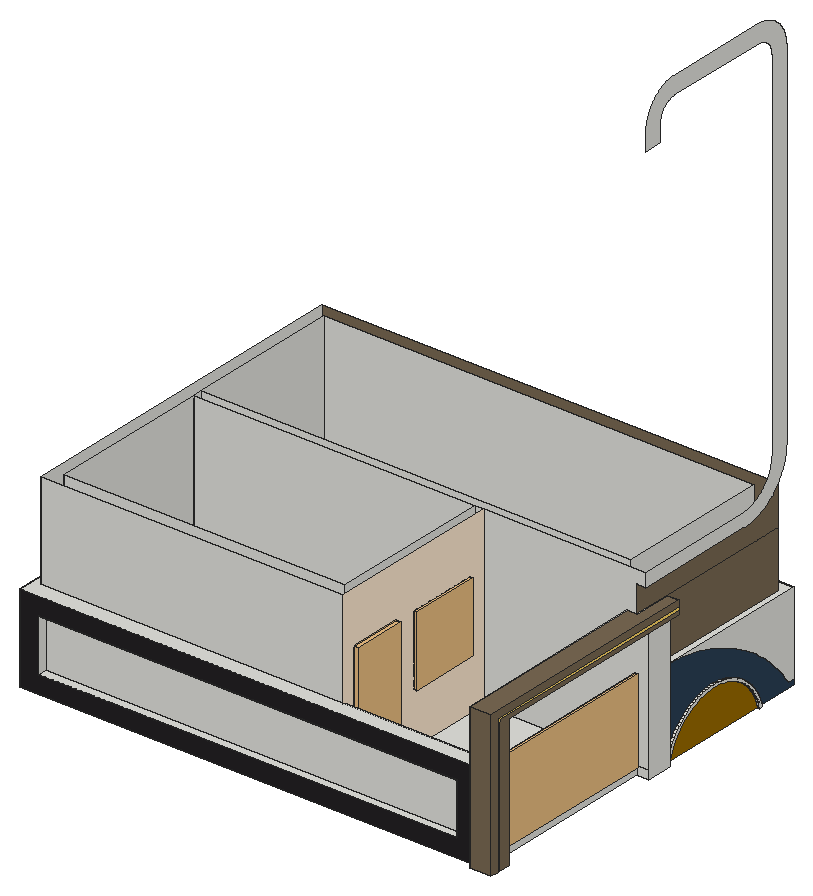
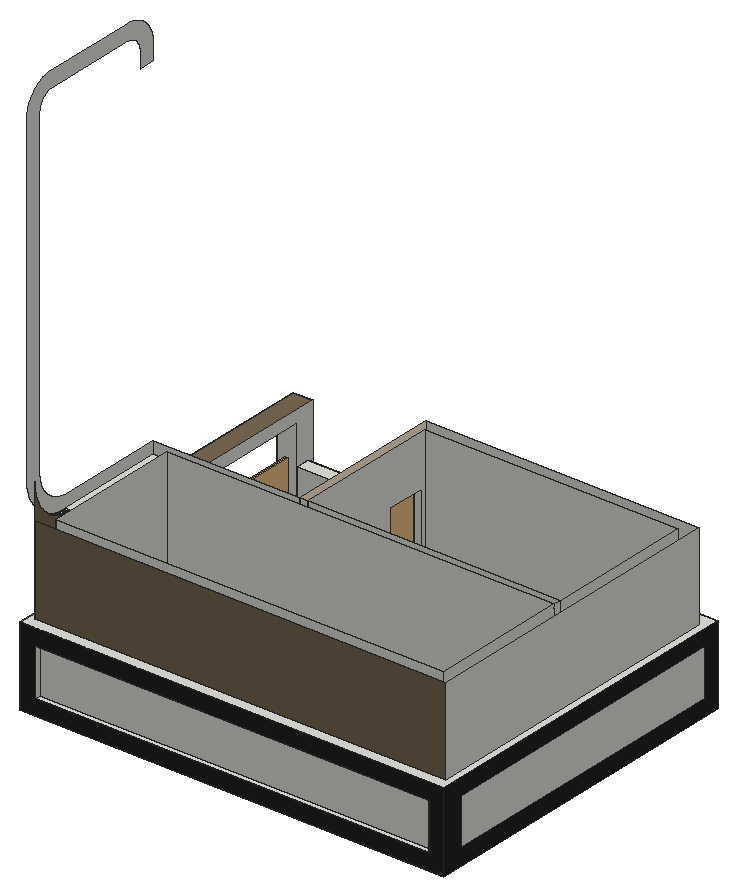
# SketchUp Ruby script. Lengths in inches.
U = 1.inch
M = Sketchup.active_model
def pt(a) = Geom::Point3d.new(a.map { |v| v * U })
def face(e, loops, mat)
  f = e.add_face(loops[0].map { |a| pt(a) })
  loops[1..].each { |l| e.add_face(l.map { |a| pt(a) }).erase! }
  f.material = f.back_material = mat if mat
  f
end
# faces: each face lists its corners as indices into pts; further lists are holes
def faces(e, pts, list, mat = nil) = list.each { |f| face(e, (f[0].is_a?(Array) ? f : [f]).map { |l| l.map { |i| pts[i] } }, mat) }
# xy, xz, yz: faces in a plane at the given z, y or x. An outline is a flat list of corners, or four numbers for a rectangle; further outlines are holes
def ring(l) = l.size == 4 ? [[l[0], l[1]], [l[2], l[1]], [l[2], l[3]], [l[0], l[3]]] : l.each_slice(2).to_a
def flat(e, list, mat, &to3) = list.each { |f| face(e, (f[0].is_a?(Array) ? f : [f]).map { |l| ring(l).map { |u, v| to3.(u, v) } }, mat) }
def xy(e, z, list, mat = nil) = flat(e, list, mat) { |x, y| [x, y, z] }
def xz(e, y, list, mat = nil) = flat(e, list, mat) { |x, z| [x, y, z] }
def yz(e, x, list, mat = nil) = flat(e, list, mat) { |y, z| [x, y, z] }
def lines(e, pts, list) = list.each { |a, b| e.add_line(pt(pts[a]), pt(pts[b])) }
# prism: a flat outline (further loops are holes) pulled along v
def prism(e, loops, v, mat = nil)
  f = face(e, loops, mat); d = Geom::Vector3d.new(v.map { |x| x * U })
  f.pushpull(f.normal.samedirection?(d) ? d.length : -d.length)
end
def box(e, o, s, mat = nil) = prism(e, [[o, [o[0] + s[0], o[1], o[2]], [o[0] + s[0], o[1] + s[1], o[2]], [o[0], o[1] + s[1], o[2]]]], [0, 0, s[2]], mat)
def at(x, y, z, deg = 0) = Geom::Transformation.translation(pt([x, y, z])) * Geom::Transformation.rotation(ORIGIN, Z_AXIS, deg.degrees)
def axes(o, x, y, z) = Geom::Transformation.new([*x, 0, *y, 0, *z, 0, *pt(o).to_a, 1])
def part(name) = M.definitions.add(name)
# library, detail: a bought-in or finely detailed component or shape, given as its bounding box
def library(name, o, s) = part(name).tap { |d| box(d.entities, o, s) }
def detail(e, o, s) = box(e.add_group.entities, o, s)
def put(e, d, t, mat = nil) = e.add_instance(d, t).tap { |i| i.material = mat if mat }
def group(e, t, mat = nil) = e.add_group.tap { |g| g.transformation = t; g.material = mat if mat }.entities
root = M.entities
M.materials.add("C03_Honey_Glow").color = [255, 234, 209]
M.materials.add("Carpet_04_1K").color = [43, 65, 85]
M.materials.add("D03_Lemon_Mist").color = [255, 216, 101]
M.materials.add("D07_Ochre_Flame").color = [153, 107, 0]
M.materials.add("Marble_07_1K").color = [36, 34, 36]
M.materials.add("Plaster_03_1K").color = [121, 105, 83]
c1 = library("porta+4",[0.2,-5.42,1.33],[46.55,4.72,83.21])
c2 = library("Modern+Gate+1",[0,0,0],[118.11,1.97,78.74])
c3 = library("mesh-165",[-1596.32,-2661.67,-39.91],[1702.88,1739.15,82.5])
c4 = part("Group15")
put(c4.entities,c3,at(294.66,859.51,3.5))
xy(root,0,[[310.73,0,325.5,15],[0,4.5,0,263.5,321.5,263.5,321.5,234.4,323.5,234.4,323.5,232.4,321.5,232.4,321.5,155,323.5,155,323.5,153,325.5,153,325.5,135,317.5,135,317.5,15,310.73,15,310.73,4.5]])
xy(root,6,[[212.5,15,317.5,15,317.5,135,308.5,135,308.5,24,212.5,24],[14.5,24,206.5,135],[212.5,24,308.5,135],[14.5,141,308.5,246]])
xy(root,9,[[206.5,27,212.5,57]])
xy(root,12,[[13,4.5,298.73,10.5],[0,16.5,1,247.5],[12,259.5,309.5,263.5]])
xy(root,45,[[206.5,78,212.5,120]])
xy(root,48,[[13,4.5,298.73,10.5],[0,16.5,1,247.5],[12,259.5,309.5,263.5]])
xy(root,60,[[0,4.5,310.73,4.5,310.73,15,5.5,15,5.5,255,317.5,255,317.5,153,321.5,153,321.5,263.5,0,263.5]])
xy(root,87,[[206.5,27,212.5,57],[206.5,78,212.5,120]])
xy(root,89.79,[[310.73,15,325.5,135],[317.5,135,325.5,153],[317.5,153,325.5,160.64]])
xy(root,98.79,[[310.73,0,325.5,0,325.5,160.64,317.5,160.64,317.5,135,310.73,135]],"Plaster_03_1K")
xy(root,117,[[317.5,135,323.5,219]])
xz(root,0,[[310.73,0,325.5,98.79]],"Plaster_03_1K")
xz(root,4.5,[[[0,0,310.73,60],[13,12,298.73,48]]],"Marble_07_1K")
xz(root,10.5,[[13,12,298.73,48]])
xz(root,15,[[310.73,0,317.5,6],[317.5,0,317.5,6,310.73,6,310.73,89.79,325.5,89.79,325.5,0],[212.5,6,310.73,60],[5.5,60,212.5,126]])
xz(root,16.5,[[0,12,1,48]])
xz(root,24,[[14.5,6,206.5,126]])
xz(root,27,[[206.5,9,212.5,87]])
xz(root,57,[[206.5,9,212.5,87]])
xz(root,78,[[206.5,45,212.5,87]])
xz(root,120,[[206.5,45,212.5,87]])
xz(root,135,[[317.5,0,325.5,6],[14.5,6,206.5,126],[206.5,6,212.5,126],[212.5,6,325.5,6,325.5,89.79,310.73,89.79,310.73,98.79,317.5,98.79,317.5,117,323.5,117,323.5,126,212.5,126],[310.73,89.79,317.5,98.79]])
xz(root,141,[[14.5,6,308.5,126]])
xz(root,153,[[321.5,0,325.5,60],[317.5,60,325.5,89.79]])
xz(root,160.64,[[317.5,89.79,325.5,98.79]])
xz(root,246,[[14.5,6,308.5,126]])
xz(root,247.5,[[0,12,1,48]])
xz(root,255,[[5.5,60,317.5,126]],"Plaster_03_1K")
xz(root,259.5,[[12,12,309.5,48]])
xz(root,263.5,[[[0,0,321.5,60],[12,12,309.5,48]]],"Marble_07_1K")
yz(root,0,[[[4.5,0,263.5,60],[16.5,12,247.5,48]]],"Marble_07_1K")
yz(root,1,[[16.5,12,247.5,48]])
yz(root,5.5,[[15,60,255,126]])
yz(root,12,[[259.5,12,263.5,48]])
yz(root,13,[[4.5,12,10.5,48]])
yz(root,14.5,[[24,6,135,126],[135,6,141,126],[141,6,246,126]])
yz(root,206.5,[[[24,6,135,126],[27,9,57,87],[78,45,120,87]]])
yz(root,212.5,[[[24,6,60,90],[27,9,57,87]],[[75,42,123,90],[78,45,120,87]]])
yz(root,212.5,[[[15,6,24,6,24,90,60,90,60,6,135,6,135,126,15,126],[75,42,123,90]]],"C03_Honey_Glow")
yz(root,298.73,[[4.5,12,10.5,48]])
yz(root,308.5,[[141,6,246,126]])
yz(root,309.5,[[259.5,12,263.5,48]])
yz(root,310.73,[[0,0,0,98.79,135,98.79,135,89.79,15,89.79,15,60,4.5,60,4.5,0],[4.5,0,15,60]])
yz(root,317.5,[[15,0,135,6],[135,89.79,160.64,98.79]])
yz(root,317.5,[[153,60,255,60,255,98.79,160.64,98.79,160.64,89.79,153,89.79],[135,98.79,255,98.79,255,153,254.99,151.87,254.95,150.73,254.87,149.6,254.75,148.48,254.6,147.35,254.41,146.24,254.18,145.125,253.93,144.02,253.63,142.93,253.3,141.84,252.94,140.77,252.55,139.71,252.12,138.66,251.65,137.62,251.16,136.6,250.63,135.6,250.07,134.61,249.48,133.65,248.86,132.7,248.21,131.77,247.53,130.86,246.83,129.98,246.09,129.11,245.33,128.27,244.54,127.46,243.73,126.67,243,126.01,243,126,242.99,126,242.89,125.91,242.02,125.17,241.14,124.47,240.23,123.79,239.3,123.14,238.35,122.52,237.39,121.93,236.4,121.37,235.4,120.84,234.38,120.35,233.34,119.88,232.29,119.45,231.23,119.06,230.16,118.7,229.07,118.37,227.98,118.07,226.875,117.82,225.76,117.59,224.65,117.4,223.52,117.25,222.4,117.13,221.27,117.05,220.13,117.01,219,117,135,117]],"Plaster_03_1K")
yz(root,321.5,[[259.5,3.75,263.5,3.75,263.5,60,153,60,155.5,59.96,158.01,59.875,160.51,59.74,163,59.56,165.5,59.33,167.99,59.05,170.47,58.72,172.94,58.35,175.41,57.93,177.87,57.46,180.32,56.95,182.76,56.38,185.19,55.77,187.61,55.12,190.01,54.42,192.4,53.67,194.78,52.875,197.14,52.03,199.48,51.15,201.8,50.22,204.11,49.25,206.4,48.23,208.67,47.17,210.91,46.06,213.14,44.91,215.34,43.72,217.52,42.49,219.67,41.21,221.81,39.9,223.91,38.54,225.99,37.15,228.04,35.71,230.0625,34.23,232.06,32.72,234.02,31.17,235.96,29.58,237.86,27.95,239.73,26.29,241.57,24.59,243.38,22.86,245.16,21.09,246.89,19.29,248.6,17.46,250.27,15.59,251.9,13.69,253.5,11.76,255.05,9.8,256.57,7.8125,258.06,5.79]])
yz(root,321.5,[[153,0,153.59,2.15,154.3,4.26,155.11,6.33,156.04,8.36,157.07,10.33,158.21,12.25,159.44,14.11,160.77,15.89,162.2,17.6,163.71,19.24,165.31,20.79,166.99,22.25,168.74,23.63,170.57,24.91,172.46,26.08,174.41,27.16,176.41,28.13,178.46,29,180.56,29.75,182.69,30.4,184.86,30.92,187.05,31.33,189.25,31.63,191.48,31.81,193.7,31.87,195.93,31.81,198.15,31.63,200.36,31.33,202.55,30.92,204.71,30.4,206.84,29.75,208.94,29,210.99,28.13,213,27.16,214.95,26.08,216.84,24.91,218.66,23.63,220.42,22.25,222.1,20.79,223.69,19.24,225.21,17.6,226.63,15.89,227.96,14.11,229.2,12.25,230.33,10.33,231.37,8.36,232.29,6.33,233.11,4.26,233.8125,2.15,234.4,0,263.5,0,263.5,3.75,259.5,3.75,258.06,5.79,256.57,7.8125,255.05,9.8,253.5,11.76,251.9,13.69,250.27,15.59,248.6,17.46,246.89,19.29,245.16,21.09,243.38,22.86,241.57,24.59,239.73,26.29,237.86,27.95,235.96,29.58,234.02,31.17,232.06,32.72,230.0625,34.23,228.04,35.71,225.99,37.15,223.91,38.54,221.81,39.9,219.67,41.21,217.52,42.49,215.34,43.72,213.14,44.91,210.91,46.06,208.67,47.17,206.4,48.23,204.11,49.25,201.8,50.22,199.48,51.15,197.14,52.03,194.78,52.875,192.4,53.67,190.01,54.42,187.61,55.12,185.19,55.77,182.76,56.38,180.32,56.95,177.87,57.46,175.41,57.93,172.94,58.35,170.47,58.72,167.99,59.05,165.5,59.33,163,59.56,160.51,59.74,158.01,59.875,155.5,59.96,153,60]],"Carpet_04_1K")
yz(root,321.5,[[155,0,232.4,0,231.84,2.04,231.17,4.05,230.39,6.02,229.51,7.9375,228.52,9.8125,227.44,11.63,226.27,13.39,225,15.09,223.65,16.72,222.21,18.27,220.6875,19.74,219.09,21.13,217.42,22.43,215.6875,23.65,213.89,24.77,212.04,25.79,210.13,26.71,208.18,27.53,206.19,28.25,204.16,28.86,202.11,29.36,200.03,29.75,197.93,30.03,195.82,30.2,193.7,30.25,191.59,30.2,189.48,30.03,187.38,29.75,185.3,29.36,183.24,28.86,181.21,28.25,179.22,27.53,177.27,26.71,175.37,25.79,173.51,24.77,171.72,23.65,169.98,22.43,168.32,21.13,166.72,19.74,165.2,18.27,163.76,16.72,162.4,15.09,161.14,13.39,159.96,11.63,158.88,9.8125,157.9,7.9375,157.02,6.02,156.24,4.05,155.57,2.04]],"D07_Ochre_Flame")
yz(root,323.5,[[153,0,155,0,155.57,2.04,156.24,4.05,157.02,6.02,157.9,7.9375,158.88,9.8125,159.96,11.63,161.14,13.39,162.4,15.09,163.76,16.72,165.2,18.27,166.72,19.74,168.32,21.13,169.98,22.43,171.72,23.65,173.51,24.77,175.37,25.79,177.27,26.71,179.22,27.53,181.21,28.25,183.24,28.86,185.3,29.36,187.38,29.75,189.48,30.03,191.59,30.2,193.7,30.25,195.82,30.2,197.93,30.03,200.03,29.75,202.11,29.36,204.16,28.86,206.19,28.25,208.18,27.53,210.13,26.71,212.04,25.79,213.89,24.77,215.6875,23.65,217.42,22.43,219.09,21.13,220.6875,19.74,222.21,18.27,223.65,16.72,225,15.09,226.27,13.39,227.44,11.63,228.52,9.8125,229.51,7.9375,230.39,6.02,231.17,4.05,231.84,2.04,232.4,0,234.4,0,233.8125,2.15,233.11,4.26,232.29,6.33,231.37,8.36,230.33,10.33,229.2,12.25,227.96,14.11,226.63,15.89,225.21,17.6,223.69,19.24,222.1,20.79,220.42,22.25,218.66,23.63,216.84,24.91,214.95,26.08,213,27.16,210.99,28.13,208.94,29,206.84,29.75,204.71,30.4,202.55,30.92,200.36,31.33,198.15,31.63,195.93,31.81,193.7,31.87,191.48,31.81,189.25,31.63,187.05,31.33,184.86,30.92,182.69,30.4,180.56,29.75,178.46,29,176.41,28.13,174.41,27.16,172.46,26.08,170.57,24.91,168.74,23.63,166.99,22.25,165.31,20.79,163.71,19.24,162.2,17.6,160.77,15.89,159.44,14.11,158.21,12.25,157.07,10.33,156.04,8.36,155.11,6.33,154.3,4.26,153.59,2.15],[135,117,219,117,220.13,117.01,221.27,117.05,222.4,117.13,223.52,117.25,224.65,117.4,225.76,117.59,226.875,117.82,227.98,118.07,229.07,118.37,230.16,118.7,231.23,119.06,232.29,119.45,233.34,119.88,234.38,120.35,235.4,120.84,236.4,121.37,237.39,121.93,238.35,122.52,239.3,123.14,240.23,123.79,241.14,124.47,242.02,125.17,242.89,125.91,242.99,126,243,126.01,243.73,126.67,244.54,127.46,245.33,128.27,246.09,129.11,246.83,129.98,247.53,130.86,248.21,131.77,248.86,132.7,249.48,133.65,250.07,134.61,250.63,135.6,251.16,136.6,251.65,137.62,252.12,138.66,252.55,139.71,252.94,140.77,253.3,141.84,253.63,142.93,253.93,144.02,254.18,145.125,254.41,146.24,254.6,147.35,254.75,148.48,254.87,149.6,254.95,150.73,254.99,151.87,255,153,255,396,254.99,396.76,254.96,397.51,254.91,398.26,254.83,399.01,254.73,399.76,254.6,400.51,254.45,401.25,254.28,401.98,254.08,402.71,253.86,403.4375,253.62,404.15,253.36,404.86,253.07,405.56,252.76,406.25,252.43,406.93,252.08,407.6,251.85,408,251.71,408.25,251.3125,408.9,250.9,409.53,250.47,410.15,250.01,410.75,249.54,411.34,249.05,411.92,248.54,412.48,248.02,413.02,247.48,413.54,247,413.98,246.92,414.05,246.34,414.54,245.75,415.01,245.15,415.47,244.53,415.9,243.9,416.3125,243.25,416.71,242.6,417.08,241.93,417.43,241.25,417.76,240.56,418.07,239.86,418.36,239.15,418.62,238.4375,418.86,237.71,419.08,236.98,419.28,236.25,419.45,235.51,419.6,234.76,419.73,234.01,419.83,233.26,419.91,232.51,419.96,231.76,419.99,231,420,159,420,158.25,419.97,157.5,419.92,156.76,419.85,156.01,419.76,155.27,419.64,154.53,419.5,153.8,419.34,153.08,419.15,152.35,418.94,151.64,418.71,150.93,418.46,150.24,418.19,149.55,417.9,148.86,417.58,148.19,417.25,147.53,416.89,146.89,416.52,146.25,416.12,145.625,415.7,145.01,415.27,144.41,414.82,143.83,414.35,143.26,413.86,142.71,413.35,142.17,412.83,141.65,412.29,141.14,411.74,140.65,411.17,140.18,410.59,139.73,409.99,139.3,409.375,138.88,408.75,138.48,408.11,138.11,407.47,137.75,406.81,137.42,406.14,137.1,405.45,136.81,404.76,136.54,404.07,136.29,403.36,136.06,402.65,135.85,401.92,135.66,401.2,135.5,400.47,135.36,399.73,135.24,398.99,135.15,398.24,135.08,397.5,135.03,396.75,135,396,135,384,147,384,147,396,147.01,396.375,147.03,396.75,147.11,397.5,147.17,397.87,147.24,398.24,147.32,398.61,147.41,398.97,147.51,399.33,147.625,399.6875,147.75,400.04,147.88,400.39,148.03,400.74,148.1875,401.08,148.35,401.42,148.53,401.75,148.72,402.07,149.12,402.71,149.34,403.01,149.57,403.3125,149.8,403.61,150.3,404.17,150.56,404.44,150.83,404.7,151.39,405.2,151.6875,405.43,151.99,405.66,152.29,405.88,152.93,406.28,153.25,406.47,153.58,406.65,153.92,406.8125,154.26,406.97,154.61,407.12,154.96,407.25,155.3125,407.375,155.67,407.49,156.03,407.59,156.39,407.68,156.76,407.76,157.13,407.83,157.5,407.89,158.25,407.97,158.625,407.99,159,408,231.38,408,231.76,407.98,232.13,407.96,232.51,407.92,232.88,407.87,233.26,407.81,233.63,407.74,234,407.65,234.72,407.45,235.08,407.33,235.4375,407.19,235.79,407.05,236.13,406.9,236.81,406.56,237.14,406.37,237.78,405.97,238.09,405.75,238.39,405.52,238.6875,405.29,238.97,405.04,239.25,404.79,239.53,404.53,239.79,404.25,240.04,403.97,240.29,403.6875,240.52,403.39,240.75,403.09,240.97,402.78,241.37,402.14,241.56,401.81,241.9,401.13,242.05,400.79,242.19,400.4375,242.33,400.08,242.45,399.72,242.65,399,242.74,398.63,242.81,398.26,242.87,397.88,242.92,397.51,242.96,397.13,242.98,396.76,243,396.38,243,153,243.02,152.2,243.02,151.4,243,150.75,243,150.6,242.94,149.81,242.87,149.01,242.77,148.22,242.64,147.43,242.5,146.64,242.32,145.86,242.125,145.09,241.91,144.32,241.66,143.56,241.39,142.8,241.1,142.06,240.79,141.32,240.45,140.6,240.1,139.88,239.72,139.18,239.32,138.49,238.89,137.8125,238.45,137.15,237.99,136.49,237.5,135.86,237,135.24,236.48,134.63,235.9375,134.04,235.38,133.47,234.8,132.91,234.21,132.38,233.6,131.86,232.98,131.36,232.34,130.88,231.6875,130.42,231.02,129.98,230.34,129.5625,229.64,129.17,228.9375,128.79,228.22,128.4375,227.49,128.1,226.76,127.8,226.01,127.51,225.26,127.25,224.49,127.01,223.72,126.79,222.95,126.6,222.17,126.43,221.38,126.29,220.59,126.17,219.8,126.07,219,126,135,126]])
yz(root,325.5,[[135,0,153,89.79]])
yz(root,325.5,[[5.5,0,7.5,0,7.5,92.29,160.64,92.29,160.64,94.29,5.5,94.29]],"D03_Lemon_Mist")
yz(root,325.5,[[0,0,5.5,0,5.5,94.29,160.64,94.29,160.64,98.79,0,98.79],[7.5,0,15,0,15,89.79,160.64,89.79,160.64,92.29,7.5,92.29]],"Plaster_03_1K")
p = [[321.5,153.59,2.15],[321.5,153,0],[323.5,153,0],[323.5,153.59,2.15],[321.5,155,0],[321.5,155.57,2.04],
  [323.5,155.57,2.04],[323.5,155,0],[321.5,231.84,2.04],[321.5,232.4,0],[323.5,232.4,0],[323.5,231.84,2.04],
  [321.5,234.4,0],[321.5,233.8125,2.15],[323.5,233.8125,2.15],[323.5,234.4,0],[321.5,156.24,4.05],[323.5,156.24,4.05],
  [321.5,231.17,4.05],[323.5,231.17,4.05],[321.5,154.3,4.26],[323.5,154.3,4.26],[321.5,233.11,4.26],[323.5,233.11,4.26],
  [321.5,157.02,6.02],[323.5,157.02,6.02],[321.5,230.39,6.02],[323.5,230.39,6.02],[321.5,155.11,6.33],[323.5,155.11,6.33],
  [321.5,232.29,6.33],[323.5,232.29,6.33],[321.5,157.9,7.9375],[323.5,157.9,7.9375],[321.5,229.51,7.9375],[323.5,229.51,7.9375],
  [321.5,156.04,8.36],[323.5,156.04,8.36],[321.5,231.37,8.36],[323.5,231.37,8.36],[321.5,158.88,9.8125],[323.5,158.88,9.8125],
  [321.5,228.52,9.8125],[323.5,228.52,9.8125],[321.5,157.07,10.33],[323.5,157.07,10.33],[321.5,230.33,10.33],[323.5,230.33,10.33],
  [321.5,159.96,11.63],[323.5,159.96,11.63],[321.5,227.44,11.63],[323.5,227.44,11.63],[321.5,158.21,12.25],[323.5,158.21,12.25],
  [321.5,229.2,12.25],[323.5,229.2,12.25],[321.5,161.14,13.39],[323.5,161.14,13.39],[321.5,226.27,13.39],[323.5,226.27,13.39],
  [321.5,159.44,14.11],[323.5,159.44,14.11],[321.5,227.96,14.11],[323.5,227.96,14.11],[321.5,162.4,15.09],[323.5,162.4,15.09],
  [321.5,225,15.09],[323.5,225,15.09],[321.5,160.77,15.89],[323.5,160.77,15.89],[321.5,226.63,15.89],[323.5,226.63,15.89],
  [321.5,163.76,16.72],[323.5,163.76,16.72],[321.5,223.65,16.72],[323.5,223.65,16.72],[321.5,162.2,17.6],[323.5,162.2,17.6],
  [321.5,225.21,17.6],[323.5,225.21,17.6],[321.5,165.2,18.27],[323.5,165.2,18.27],[321.5,222.21,18.27],[323.5,222.21,18.27],
  [321.5,163.71,19.24],[323.5,163.71,19.24],[321.5,223.69,19.24],[323.5,223.69,19.24],[321.5,166.72,19.74],[323.5,166.72,19.74],
  [321.5,220.6875,19.74],[323.5,220.6875,19.74],[321.5,165.31,20.79],[323.5,165.31,20.79],[321.5,222.1,20.79],[323.5,222.1,20.79],
  [321.5,168.32,21.13],[323.5,168.32,21.13],[321.5,219.09,21.13],[323.5,219.09,21.13],[321.5,166.99,22.25],[323.5,166.99,22.25],
  [321.5,220.42,22.25],[323.5,220.42,22.25],[321.5,169.98,22.43],[323.5,169.98,22.43],[321.5,217.42,22.43],[323.5,217.42,22.43],
  [321.5,168.74,23.63],[323.5,168.74,23.63],[321.5,218.66,23.63],[323.5,218.66,23.63],[321.5,171.72,23.65],[323.5,171.72,23.65],
  [321.5,215.6875,23.65],[323.5,215.6875,23.65],[321.5,170.57,24.91],[323.5,170.57,24.91],[321.5,173.51,24.77],[323.5,173.51,24.77],
  [321.5,213.89,24.77],[323.5,213.89,24.77],[321.5,216.84,24.91],[323.5,216.84,24.91],[321.5,175.37,25.79],[323.5,175.37,25.79],
  [321.5,212.04,25.79],[323.5,212.04,25.79],[321.5,172.46,26.08],[323.5,172.46,26.08],[321.5,214.95,26.08],[323.5,214.95,26.08],
  [321.5,177.27,26.71],[323.5,177.27,26.71],[321.5,210.13,26.71],[323.5,210.13,26.71],[321.5,174.41,27.16],[323.5,174.41,27.16],
  [321.5,213,27.16],[323.5,213,27.16],[321.5,179.22,27.53],[323.5,179.22,27.53],[321.5,208.18,27.53],[323.5,208.18,27.53],
  [321.5,176.41,28.13],[323.5,176.41,28.13],[321.5,210.99,28.13],[323.5,210.99,28.13],[321.5,181.21,28.25],[323.5,181.21,28.25],
  [321.5,206.19,28.25],[323.5,206.19,28.25],[321.5,178.46,29],[323.5,178.46,29],[321.5,208.94,29],[323.5,208.94,29],
  [321.5,183.24,28.86],[323.5,183.24,28.86],[321.5,204.16,28.86],[323.5,204.16,28.86],[321.5,185.3,29.36],[323.5,185.3,29.36],
  [321.5,202.11,29.36],[323.5,202.11,29.36],[321.5,180.56,29.75],[323.5,180.56,29.75],[321.5,206.84,29.75],[323.5,206.84,29.75],
  [321.5,187.38,29.75],[323.5,187.38,29.75],[321.5,200.03,29.75],[323.5,200.03,29.75],[321.5,189.48,30.03],[323.5,189.48,30.03],
  [321.5,197.93,30.03],[323.5,197.93,30.03],[321.5,182.69,30.4],[323.5,182.69,30.4],[321.5,204.71,30.4],[323.5,204.71,30.4],
  [321.5,191.59,30.2],[323.5,191.59,30.2],[321.5,195.82,30.2],[323.5,195.82,30.2],[321.5,193.7,30.25],[323.5,193.7,30.25],
  [321.5,184.86,30.92],[323.5,184.86,30.92],[321.5,202.55,30.92],[323.5,202.55,30.92],[321.5,187.05,31.33],[323.5,187.05,31.33],
  [321.5,200.36,31.33],[323.5,200.36,31.33],[321.5,189.25,31.63],[323.5,189.25,31.63],[321.5,198.15,31.63],[323.5,198.15,31.63],
  [321.5,191.48,31.81],[323.5,191.48,31.81],[321.5,195.93,31.81],[323.5,195.93,31.81],[321.5,193.7,31.87],[323.5,193.7,31.87],
  [317.5,219,117],[317.5,220.13,117.01],[323.5,220.13,117.01],[323.5,219,117],[317.5,221.27,117.05],[323.5,221.27,117.05],
  [317.5,222.4,117.13],[323.5,222.4,117.13],[317.5,223.52,117.25],[323.5,223.52,117.25],[317.5,224.65,117.4],[323.5,224.65,117.4],
  [317.5,225.76,117.59],[323.5,225.76,117.59],[317.5,226.875,117.82],[323.5,226.875,117.82],[317.5,227.98,118.07],[323.5,227.98,118.07],
  [317.5,229.07,118.37],[323.5,229.07,118.37],[317.5,230.16,118.7],[323.5,230.16,118.7],[317.5,231.23,119.06],[323.5,231.23,119.06],
  [317.5,232.29,119.45],[323.5,232.29,119.45],[317.5,233.34,119.88],[323.5,233.34,119.88],[317.5,234.38,120.35],[323.5,234.38,120.35],
  [317.5,235.4,120.84],[323.5,235.4,120.84],[317.5,236.4,121.37],[323.5,236.4,121.37],[317.5,237.39,121.93],[323.5,237.39,121.93],
  [317.5,238.35,122.52],[323.5,238.35,122.52],[317.5,239.3,123.14],[323.5,239.3,123.14],[317.5,240.23,123.79],[323.5,240.23,123.79],
  [317.5,241.14,124.47],[323.5,241.14,124.47],[317.5,242.02,125.17],[323.5,242.02,125.17],[317.5,242.89,125.91],[323.5,242.89,125.91],
  [321.5,155,1],[321.5,232.4,1]]
faces(root,p,[[0,1,2,3],[4,5,6,7],[8,9,10,11],[12,13,14,15],[5,16,17,6],[18,8,11,19],[20,0,3,21],[13,22,23,14],
  [16,24,25,17],[26,18,19,27],[28,20,21,29],[22,30,31,23],[24,32,33,25],[34,26,27,35],[36,28,29,37],[30,38,39,31],
  [32,40,41,33],[42,34,35,43],[44,36,37,45],[38,46,47,39],[40,48,49,41],[50,42,43,51],[52,44,45,53],[46,54,55,47],
  [48,56,57,49],[58,50,51,59],[60,52,53,61],[54,62,63,55],[56,64,65,57],[66,58,59,67],[68,60,61,69],[62,70,71,63],
  [64,72,73,65],[74,66,67,75],[76,68,69,77],[70,78,79,71],[72,80,81,73],[82,74,75,83],[84,76,77,85],[78,86,87,79],
  [80,88,89,81],[90,82,83,91],[92,84,85,93],[86,94,95,87],[88,96,97,89],[98,90,91,99],[100,92,93,101],[94,102,103,95],
  [96,104,105,97],[106,98,99,107],[108,100,101,109],[102,110,111,103],[104,112,113,105],[114,106,107,115],[116,108,109,117],[112,118,119,113],
  [120,114,115,121],[110,122,123,111],[118,124,125,119],[126,120,121,127],[128,116,117,129],[122,130,131,123],[124,132,133,125],[134,126,127,135],
  [136,128,129,137],[130,138,139,131],[132,140,141,133],[142,134,135,143],[144,136,137,145],[138,146,147,139],[140,148,149,141],[150,142,143,151],
  [152,144,145,153],[146,154,155,147],[148,156,157,149],[158,150,151,159],[156,160,161,157],[162,158,159,163],[164,152,153,165],[154,166,167,155],
  [160,168,169,161],[170,162,163,171],[168,172,173,169],[174,170,171,175],[176,164,165,177],[166,178,179,167],[172,180,181,173],[182,174,175,183],
  [180,184,185,181],[184,182,183,185],[186,176,177,187],[178,188,189,179],[190,186,187,191],[188,192,193,189],[194,190,191,195],[192,196,197,193],
  [198,194,195,199],[196,200,201,197],[202,198,199,203],[200,202,203,201],[204,205,206,207],[205,208,209,206],[208,210,211,209],[210,212,213,211],
  [212,214,215,213],[214,216,217,215],[216,218,219,217],[218,220,221,219],[220,222,223,221],[222,224,225,223],[224,226,227,225],[226,228,229,227],
  [228,230,231,229],[230,232,233,231],[232,234,235,233],[234,236,237,235],[236,238,239,237],[238,240,241,239],[240,242,243,241],[242,244,245,243],
  [244,246,247,245],[246,248,249,247],[248,250,251,249]])
lines(root,p,[[252,4],[9,253]])
put(root,c1,axes([211.97,23.76,4.64],[0,0.7752,0],[-0.76,0,0],[0,0,1.0197]))
put(root,c2,axes([319.47,15,6],[0,1,0],[-1,0,0],[0,0,0.73]))
put(root,c4,axes([213.77,86.28,91.74],[0,-0.02811,0],[0,0,0.02756],[-0.02756,0,0]))
